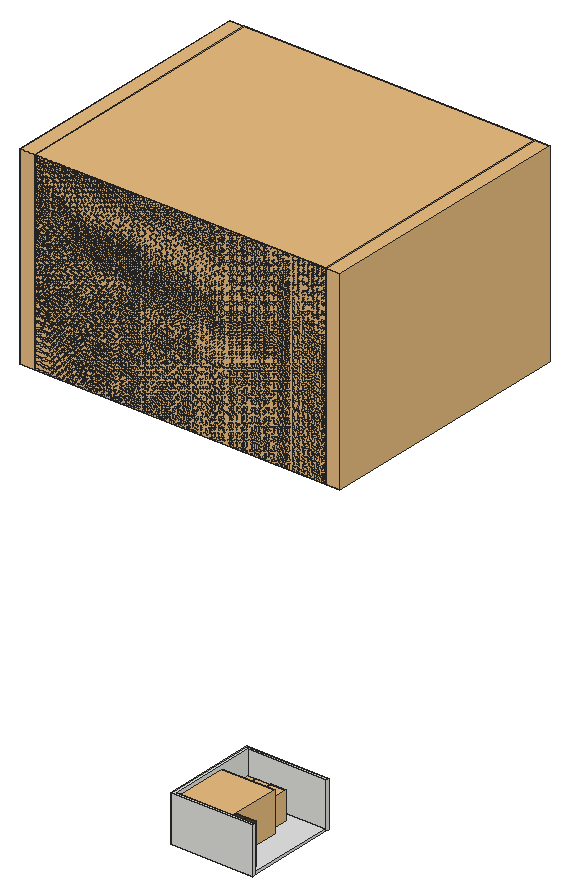
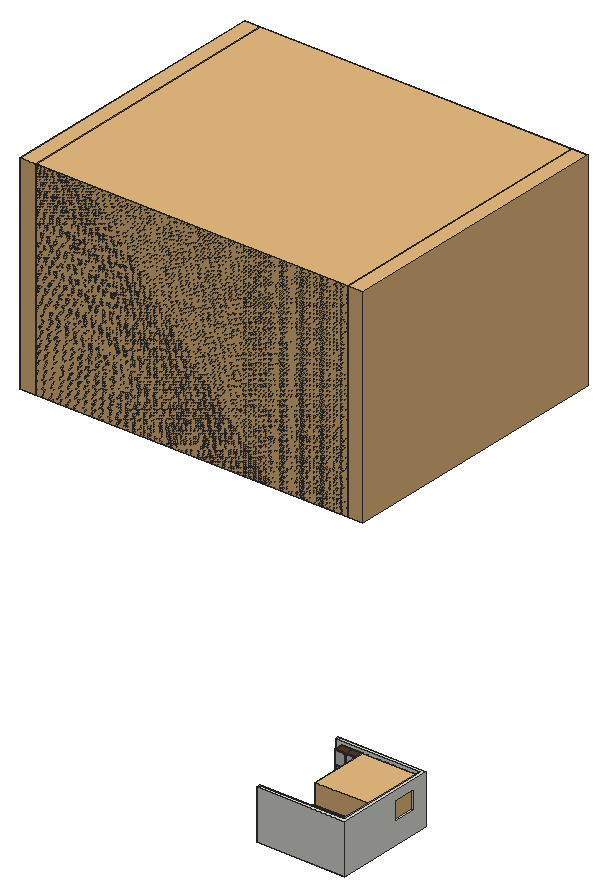
# SketchUp Ruby script. Lengths in inches.
U = 1.inch
M = Sketchup.active_model
def pt(a) = Geom::Point3d.new(a.map { |v| v * U })
def face(e, loops, mat)
  f = e.add_face(loops[0].map { |a| pt(a) })
  loops[1..].each { |l| e.add_face(l.map { |a| pt(a) }).erase! }
  f.material = f.back_material = mat if mat
  f
end
# faces: each face lists its corners as indices into pts; further lists are holes
def faces(e, pts, list, mat = nil) = list.each { |f| face(e, (f[0].is_a?(Array) ? f : [f]).map { |l| l.map { |i| pts[i] } }, mat) }
# xy, xz, yz: faces in a plane at the given z, y or x. An outline is a flat list of corners, or four numbers for a rectangle; further outlines are holes
def ring(l) = l.size == 4 ? [[l[0], l[1]], [l[2], l[1]], [l[2], l[3]], [l[0], l[3]]] : l.each_slice(2).to_a
def flat(e, list, mat, &to3) = list.each { |f| face(e, (f[0].is_a?(Array) ? f : [f]).map { |l| ring(l).map { |u, v| to3.(u, v) } }, mat) }
def xy(e, z, list, mat = nil) = flat(e, list, mat) { |x, y| [x, y, z] }
def xz(e, y, list, mat = nil) = flat(e, list, mat) { |x, z| [x, y, z] }
def yz(e, x, list, mat = nil) = flat(e, list, mat) { |y, z| [x, y, z] }
def lines(e, pts, list) = list.each { |a, b| e.add_line(pt(pts[a]), pt(pts[b])) }
# prism: a flat outline (further loops are holes) pulled along v
def prism(e, loops, v, mat = nil)
  f = face(e, loops, mat); d = Geom::Vector3d.new(v.map { |x| x * U })
  f.pushpull(f.normal.samedirection?(d) ? d.length : -d.length)
end
def box(e, o, s, mat = nil) = prism(e, [[o, [o[0] + s[0], o[1], o[2]], [o[0] + s[0], o[1] + s[1], o[2]], [o[0], o[1] + s[1], o[2]]]], [0, 0, s[2]], mat)
def at(x, y, z, deg = 0) = Geom::Transformation.translation(pt([x, y, z])) * Geom::Transformation.rotation(ORIGIN, Z_AXIS, deg.degrees)
def axes(o, x, y, z) = Geom::Transformation.new([*x, 0, *y, 0, *z, 0, *pt(o).to_a, 1])
def part(name) = M.definitions.add(name)
# library, detail: a bought-in or finely detailed component or shape, given as its bounding box
def library(name, o, s) = part(name).tap { |d| box(d.entities, o, s) }
def detail(e, o, s) = box(e.add_group.entities, o, s)
def put(e, d, t, mat = nil) = e.add_instance(d, t).tap { |i| i.material = mat if mat }
def group(e, t, mat = nil) = e.add_group.tap { |g| g.transformation = t; g.material = mat if mat }.entities
root = M.entities
M.materials.add("1466 AP 9476 Soft Whisper").color = [230, 233, 224]
M.materials.add("1472 AP 9469 Black Sea").color = [67, 75, 78]
M.materials.add("1513 AP K108 Rose Silver-N").color = [202, 201, 205]
M.materials.add("[Carrera Marble]").color = [207, 207, 207]
M.materials.add("[Granite Light Gray]").color = [49, 48, 47]
M.materials.add("[Marble Carrara Gold Floor Tile]").color = [229, 229, 229]
M.materials.add("[Translucent Glass Blue]").color = [163, 215, 254]
M.materials["[Translucent Glass Blue]"].alpha = 0.5
M.materials.add("[Translucent Glass Gray]").color = [128, 128, 128]
M.materials["[Translucent Glass Gray]"].alpha = 0.5
M.materials.add("[Wood Veneer 01]").color = [83, 56, 38]
M.materials.add("[Wood Veneer 01]1").color = [74, 43, 22]
M.materials.add("froliti-pizza_ddn").color = [170, 170, 170]
c1 = library("Group\#61",[-3.28,0,-3.2],[6.56,11.56,7.1])
c2 = library("Group1\#6",[-3.97,-4.36,4.58],[7.94,7.57,1.92])
c3 = library("Group2\#4",[-28.125,-19.52,30.85],[56.26,48.19,42.76])
c4 = part("215693")
put(c4.entities,c1,axes([0,0,0],[6.23163,0,0],[0,0,6.44624],[0,-6.23163,0]))
put(c4.entities,c2,axes([0,0.01,17.77],[2.3609,0,0],[0,2.52448,0],[0,0,1.96338]))
put(c4.entities,c3,axes([0.01,0.44,706.86],[14.88915,0,0],[0,14.88915,0],[0,0,12.38215]))
c5 = library("Object02",[-606.68,-655.71,-190.21],[1149.33,653.61,1636.06])
c6 = part("skp42")
put(c6.entities,c5,at(0,0,0))
c7 = part("Senza")
put(c7.entities,c6,at(-166.13,607.08,194.25))
c8 = library("French door refrigerator",[0,0,0],[35.5,29.25,69.5])
c9 = part("9")
box(c9.entities,[0,-0.25,-0.25],[0.5,26,33.5])
c10 = library("Potted Plant",[-13.58,-10.04,0],[38.83,39.25,67.18])
c11 = library("Group\#46",[0,0,-58.43],[152.74,148.09,107])
c12 = library("Group\#6",[0,0,0],[0.5,124,34])
c13 = part("4")
box(c13.entities,[-0.2,0,0],[0.2,23.45,29.875],"[Translucent Glass Gray]")
c14 = part("2")
xy(c14.entities,-0.25,[[-1,-0.25,0,25.45],[-1,25.55,0,51.25]])
xy(c14.entities,1,[[-1,1,0,24.2],[-1,26.8,0,50]])
xy(c14.entities,30.875,[[-1,1,0,24.2],[-1,26.8,0,50]])
xy(c14.entities,32.125,[[-1,-0.25,0,25.45],[-1,25.55,0,51.25]])
xz(c14.entities,-0.25,[[-1,-0.25,0,32.125]])
xz(c14.entities,1,[[-1,1,0,30.875]])
xz(c14.entities,24.2,[[-1,1,0,30.875]])
xz(c14.entities,25.45,[[-1,-0.25,0,32.125]])
xz(c14.entities,25.55,[[-1,-0.25,0,32.125]])
xz(c14.entities,26.8,[[-1,1,0,30.875]])
xz(c14.entities,50,[[-1,1,0,30.875]])
xz(c14.entities,51.25,[[-1,-0.25,0,32.125]])
yz(c14.entities,-1,[[[-0.25,-0.25,25.45,32.125],[1,1,24.2,30.875]],[[25.55,-0.25,51.25,32.125],[26.8,1,50,30.875]]])
yz(c14.entities,0,[[[-0.25,-0.25,25.45,32.125],[1,1,24.2,30.875]],[[25.55,-0.25,51.25,32.125],[26.8,1,50,30.875]]])
p = [[0,25.45,0],[0,25.55,0],[0,25.55,31.875],[0,25.45,31.875]]
lines(c14.entities,p,[[0,1],[2,3]])
g1 = group(c14.entities,at(-0.5625,1,1))
put(g1,c13,axes([0.2,25.8,0],[1,0,0],[0,0.98934,0],[0,0,1]))
put(g1,c13,axes([0.2,0,0],[1,0,0],[0,0.98934,0],[0,0,1]))
c15 = part("5")
box(c15.entities,[0,-0.25,-0.25],[0.5,45,11.6875])
c16 = part("6")
box(c16.entities,[0,-0.25,-0.25],[0.5,45,15.9375])
c17 = library("ACCESS \#28",[0,0,-0.01],[22.01,8.97,21.09])
c18 = library("\#1",[-189.34,-482.08,-290.58],[543.74,599.14,350.96])
c19 = part("Mixer\#1")
put(c19.entities,c18,at(-26.63,749.7,289.625))
c20 = part("תנור פולגור")
g2 = group(c20.entities,at(76.05,-2.36,7.75))
xy(g2,0,[[0.17,2.76,23.79,26.38]])
xy(g2,0,[[0,2.36,23.79,2.76]],"froliti-pizza_ddn")
xy(g2,0.23,[[0,2.34,23.79,2.76]],"froliti-pizza_ddn")
xy(g2,4.32,[[0.67,2.34,22.79,2.37]],"froliti-pizza_ddn")
xy(g2,14.64,[[0.67,2.34,22.79,2.37]],"froliti-pizza_ddn")
xy(g2,17.26,[[1.26,0,1.26,2.34,1.98,2.34,1.98,0.55,21.35,0.55,21.35,2.34,22.05,2.34,22.05,0]],"froliti-pizza_ddn")
xy(g2,17.89,[[1.26,0,22.05,0,22.05,2.34,21.35,2.34,21.35,0.55,1.98,0.55,1.98,2.34,1.26,2.34]],"froliti-pizza_ddn")
xy(g2,18.76,[[0,2.34,23.79,2.76]],"froliti-pizza_ddn")
xy(g2,19.05,[[0,2.36,0,2.76,0.17,2.76],[0,2.36,0.17,2.76,23.79,2.76,23.79,2.36]],"froliti-pizza_ddn")
xy(g2,23.62,[[0.17,2.76,23.79,26.38]])
xz(g2,0,[[1.26,17.26,22.05,17.89]],"froliti-pizza_ddn")
xz(g2,0.55,[[1.98,17.26,21.35,17.89]],"froliti-pizza_ddn")
xz(g2,2.34,[[[0,0.23,23.79,18.76],[0.67,4.32,22.79,14.64],[1.26,17.26,1.98,17.89],[21.35,17.26,22.05,17.89]]],"froliti-pizza_ddn")
xz(g2,2.36,[[[0,19.05,23.79,23.66],[3.23,19.74,20.3125,23.01]],[3.23,19.74,20.3125,23.01]],"froliti-pizza_ddn")
xz(g2,2.37,[[0.67,4.32,22.79,14.64]],"froliti-pizza_ddn")
xz(g2,2.76,[[0,0,0.17,0.23],[0,0.23,0.17,18.76],[0.17,0.23,23.79,18.76],[0,18.76,0.17,19.05],[0.17,18.76,23.79,19.05],
  [0.17,19.05,23.79,23.62]])
xz(g2,26.38,[[0.17,0,23.79,23.62]])
yz(g2,0,[[2.34,0,2.76,0.23],[2.34,0.23,2.76,18.76]])
yz(g2,0.17,[[2.76,0,26.38,23.62]])
yz(g2,0.67,[[2.34,4.32,2.37,14.64]],"froliti-pizza_ddn")
yz(g2,1.26,[[0,17.26,2.34,17.89]],"froliti-pizza_ddn")
yz(g2,1.98,[[0.55,17.26,2.34,17.89]],"froliti-pizza_ddn")
yz(g2,21.35,[[0.55,17.26,2.34,17.89]],"froliti-pizza_ddn")
yz(g2,22.05,[[0,17.26,2.34,17.89]],"froliti-pizza_ddn")
yz(g2,22.79,[[2.34,4.32,2.37,14.64]],"froliti-pizza_ddn")
yz(g2,23.79,[[2.34,0.23,2.76,18.76],[2.76,0.23,26.38,23.62],[2.36,19.05,2.76,23.62],[2.36,23.62,2.76,23.66]])
p = [[0,2.36,19.05],[0,2.36,23.62],[0.17,2.76,23.62],[0.17,2.76,19.05],[0,2.36,23.66],[0.17,2.76,23.66]]
faces(g2,p,[[0,1,2,3],[4,5,2,1]])
c21 = part("1")
box(c21.entities,[-20,0,0],[20,51,0.39])
xy(root,-6,[[0,0,0,261,225,261,225,252,9,252,9,9,225,9,225,0]])
xy(root,0,[[9,9,9,186,134,186,134,168,25,168,25,25,156,25,156,9]])
xy(root,4,[[9,9,156,9,156,25,25,25,25,168,134,168,134,186,9,186]])
xy(root,4,[[9,9,9,186,10,186,10,184.5,134,184.5,134,186,135,186,135,162,30,162,30,30,135,30,135,9]],"[Carrera Marble]")
xy(root,5.0625,[[10,10,29,10,29,31,30,31,30,52,10,52],[31,10,43,30],[44,10,88.5,30],[89.5,10,134,30],[10,53,30,88.5],
  [10,125.5,30,161],[31,162,82,162,82,183,10,183,10,163,31,163],[83,162,134,183]],"[Carrera Marble]")
xy(root,5.0625,[[10,89.5,30,124.5]],"[Wood Veneer 01]1")
xy(root,14.0625,[[10,53,29,88.5]],"[Carrera Marble]")
xy(root,15.0625,[[10,53,29,88.5]],"[Carrera Marble]")
xy(root,16.25,[[89.5,10,134,30]],"[Carrera Marble]")
xy(root,49,[[0,39,9,102]])
xy(root,97,[[0,39,9,102]])
xy(root,120,[[0,0,225,0,225,9,9,9,9,252,225,252,225,261,0,261]])
xz(root,0,[[0,-6,225,120]])
xz(root,9,[[9,-6,225,0]])
xz(root,9,[[156,0,156,4,9,4,9,120,225,120,225,0]],"1466 AP 9476 Soft Whisper")
xz(root,9,[[9,4,135,38]],"[Carrera Marble]")
xz(root,10,[[10,5.0625,29,20.5],[31,5.0625,43,36.9375],[44,5.0625,88.5,20.5],[89.5,5.0625,134,16.25]],"[Carrera Marble]")
xz(root,25,[[25,0,156,4]],"[Granite Light Gray]")
xz(root,30,[[[30,4,135,38],[44,21.5,88.5,36.9375],[44,5.0625,88.5,20.5],[89.5,17.25,134,28.4375],[89.5,5.0625,134,16.25],[31,5.0625,43,36.9375],[89.5,29.4375,134,36.9375]]],"[Wood Veneer 01]1")
xz(root,31,[[29,5.0625,30,36.9375]],"[Carrera Marble]")
xz(root,39,[[0,49,9,97]])
xz(root,52,[[10,5.0625,30,5.0625,30,36.9375,10,36.9375,10,21.5,29,21.5,29,20.5,10,20.5]],"[Carrera Marble]")
xz(root,53,[[10,5.0625,10,14.0625,29,14.0625,29,15.0625,10,15.0625,10,36.9375,30,36.9375,30,5.0625]],"[Carrera Marble]")
xz(root,88.5,[[10,5.0625,30,5.0625,30,36.9375,10,36.9375,10,15.0625,29,15.0625,29,14.0625,10,14.0625]],"[Carrera Marble]")
xz(root,89.5,[[10,5.0625,30,20.5]],"[Wood Veneer 01]1")
xz(root,102,[[0,49,9,97]])
xz(root,124.5,[[10,5.0625,30,20.5]],"[Wood Veneer 01]1")
xz(root,125.5,[[10,5.0625,30,36.9375]],"[Carrera Marble]")
xz(root,161,[[10,5.0625,30,36.9375]],"[Carrera Marble]")
xz(root,162,[[[30,4,135,38],[31,5.0625,82,36.9375],[83,5.0625,134,36.9375]]],"[Carrera Marble]")
xz(root,163,[[10,5.0625,31,36.9375]],"[Carrera Marble]")
xz(root,168,[[25,0,134,4]],"[Granite Light Gray]")
xz(root,183,[[10,5.0625,82,36.9375],[83,5.0625,134,36.9375]],"[Carrera Marble]")
xz(root,184.5,[[10,4,134,38]],"[Carrera Marble]")
xz(root,186,[[9,4,10,38],[134,4,135,38]],"[Carrera Marble]")
xz(root,186,[[9,0,134,4]],"[Granite Light Gray]")
xz(root,252,[[9,-6,225,120]])
xz(root,261,[[0,-6,225,120]])
yz(root,0,[[[0,-6,261,120],[39,49,102,97]]])
yz(root,9,[[[9,-6,252,-6,252,120,9,120,9,4,186,4,186,0,9,0],[39,49,102,97]]],"1466 AP 9476 Soft Whisper")
yz(root,9,[[9,4,186,38]],"[Carrera Marble]")
yz(root,10,[[184.5,4,186,38],[10,5.0625,52,20.5],[53,5.0625,88.5,14.0625],[125.5,5.0625,161,36.9375],[163,5.0625,183,36.9375],
  [53,15.0625,88.5,36.9375]],"[Carrera Marble]")
yz(root,10,[[89.5,5.0625,124.5,20.5]],"[Wood Veneer 01]1")
yz(root,25,[[25,0,168,4]],"[Granite Light Gray]")
yz(root,29,[[10,5.0625,31,20.5],[53,14.0625,88.5,15.0625]],"[Carrera Marble]")
yz(root,30,[[[30,4,162,38],[53,5.0625,88.5,36.9375],[125.5,5.0625,161,36.9375],[31,5.0625,52,36.9375],[89.5,21.5,124.5,36.9375],[89.5,5.0625,124.5,20.5]]],"[Wood Veneer 01]1")
yz(root,31,[[10,5.0625,30,36.9375],[162,5.0625,163,36.9375]],"[Carrera Marble]")
yz(root,43,[[10,5.0625,30,36.9375]],"[Carrera Marble]")
yz(root,44,[[10,5.0625,30,20.5]],"[Carrera Marble]")
yz(root,82,[[162,5.0625,183,36.9375]],"[Carrera Marble]")
yz(root,83,[[162,5.0625,183,36.9375]],"[Carrera Marble]")
yz(root,88.5,[[10,5.0625,30,20.5]],"[Carrera Marble]")
yz(root,89.5,[[10,5.0625,30,16.25]],"[Carrera Marble]")
yz(root,134,[[184.5,4,186,38],[10,5.0625,30,16.25],[162,5.0625,183,36.9375]],"[Carrera Marble]")
yz(root,134,[[168,0,186,4]],"[Granite Light Gray]")
yz(root,135,[[9,4,30,38],[162,4,186,38]],"[Carrera Marble]")
yz(root,156,[[9,0,25,4]])
yz(root,225,[[0,-6,9,120],[252,-6,261,120]])
g3 = group(root,at(225,9,-6,90))
xy(g3,0,[[0,0,243,216]])
xy(g3,6,[[0,0,243,216]],"[Marble Carrara Gold Floor Tile]")
xz(g3,0,[[0,0,243,6]])
xz(g3,216,[[0,0,243,6]])
yz(g3,0,[[0,0,216,6]])
yz(g3,243,[[0,0,216,6]])
put(root,c4,at(113.75,206.17,0.01),"[Carrera Marble]")
put(root,c4,at(73.125,206.17,0.01),"[Carrera Marble]")
put(root,c7,axes([31.48,211.64,-0.13],[0,0.03318,0],[-0.03716,0,0],[0,0,0.03318]))
put(root,c8,axes([209,10,0],[-1.46479,0,0],[0,0.65065,0],[0,0,1.09353]),"[Carrera Marble]")
g4 = group(root,at(210,9,0,90),"[Carrera Marble]")
xy(g4,0,[[0,0,0,54,21,54,21,53,1,53,1,1,21,1,21,0]],"[Wood Veneer 01]")
xy(g4,76,[[1,1,21,53]],"[Wood Veneer 01]")
xy(g4,77,[[1,1,21,26.5],[1,27.5,21,53]],"[Wood Veneer 01]")
xy(g4,110,[[1,1,21,26.5],[1,27.5,21,53]],"[Wood Veneer 01]")
xy(g4,111,[[0,0,21,54]],"[Wood Veneer 01]")
xz(g4,0,[[0,0,21,111]],"[Wood Veneer 01]")
xz(g4,1,[[1,0,21,76],[1,77,21,110]],"[Wood Veneer 01]")
xz(g4,26.5,[[1,77,21,110]],"[Wood Veneer 01]")
xz(g4,27.5,[[1,77,21,110]],"[Wood Veneer 01]")
xz(g4,53,[[1,0,21,76],[1,77,21,110]],"[Wood Veneer 01]")
xz(g4,54,[[0,0,21,111]],"[Wood Veneer 01]")
yz(g4,0,[[0,0,54,111]],"[Wood Veneer 01]")
yz(g4,1,[[1,0,53,76],[1,77,26.5,110],[27.5,77,53,110]],"[Wood Veneer 01]")
yz(g4,21,[[[0,0,1,0,1,76,53,76,53,0,54,0,54,111,0,111],[27.5,77,53,110],[1,77,26.5,110]]],"[Wood Veneer 01]")
put(g4,c9,at(21,1,77),"1513 AP K108 Rose Silver-N")
put(g4,c9,at(21,27.5,77),"1513 AP K108 Rose Silver-N")
put(root,c10,axes([32.5625,234.52,0],[0,0.83,0],[-0.83,0,0],[0,0,0.83]))
put(root,c11,at(156,9,62.43,90),"1472 AP 9469 Black Sea")
put(root,c12,at(134,184.5,4,90),"[Carrera Marble]")
put(root,c14,at(82,162,5.0625,90),"[Wood Veneer 01]")
put(root,c14,at(134,162,5.0625,90),"[Wood Veneer 01]")
put(root,c15,at(134,30,5.0625,90),"1472 AP 9469 Black Sea")
put(root,c16,at(88.5,30,5.0625,90),"1472 AP 9469 Black Sea")
g5 = group(root,at(43,30,5.0625,90),"1472 AP 9469 Black Sea")
box(g5,[0,-0.25,-0.25],[0.5,12.5,32.375])
g6 = group(root,at(30,31,5.0625,90),"1472 AP 9469 Black Sea")
box(g6,[-0.25,-0.5,-0.25],[21.5,0.5,32.375])
g7 = group(root,at(30,53,5.0625,90),"1472 AP 9469 Black Sea")
box(g7,[-0.25,-0.5,-0.25],[17.95,0.5,32.375])
box(g7,[17.8,-0.5,-0.25],[17.95,0.5,32.375])
p = [[17.7,0,32.125],[17.8,0,32.125]]
lines(g7,p,[[0,1]])
put(root,c17,axes([30,102.08,5.0625],[0,0.7992,0],[-1,0,0],[0,0,0.73236]),"[Carrera Marble]")
put(root,c19,axes([17.87,122.75,5.1],[0.03626,0.0007,0],[0.00072,-0.03775,0],[0,0,0.03842]),"[Carrera Marble]")
put(root,c20,axes([29.9,10.14,-5.38],[0,1.51685,0],[-0.82878,0,0],[0,0,1.34715]),"[Carrera Marble]")
put(root,c21,axes([134,183,15.55],[0,1,0],[-1,0,0],[0,0,1.0625]),"[Translucent Glass Blue]")
put(root,c21,axes([82,183,15.55],[0,1,0],[-1.41176,0,0],[0,0,1.0625]),"[Translucent Glass Blue]")
